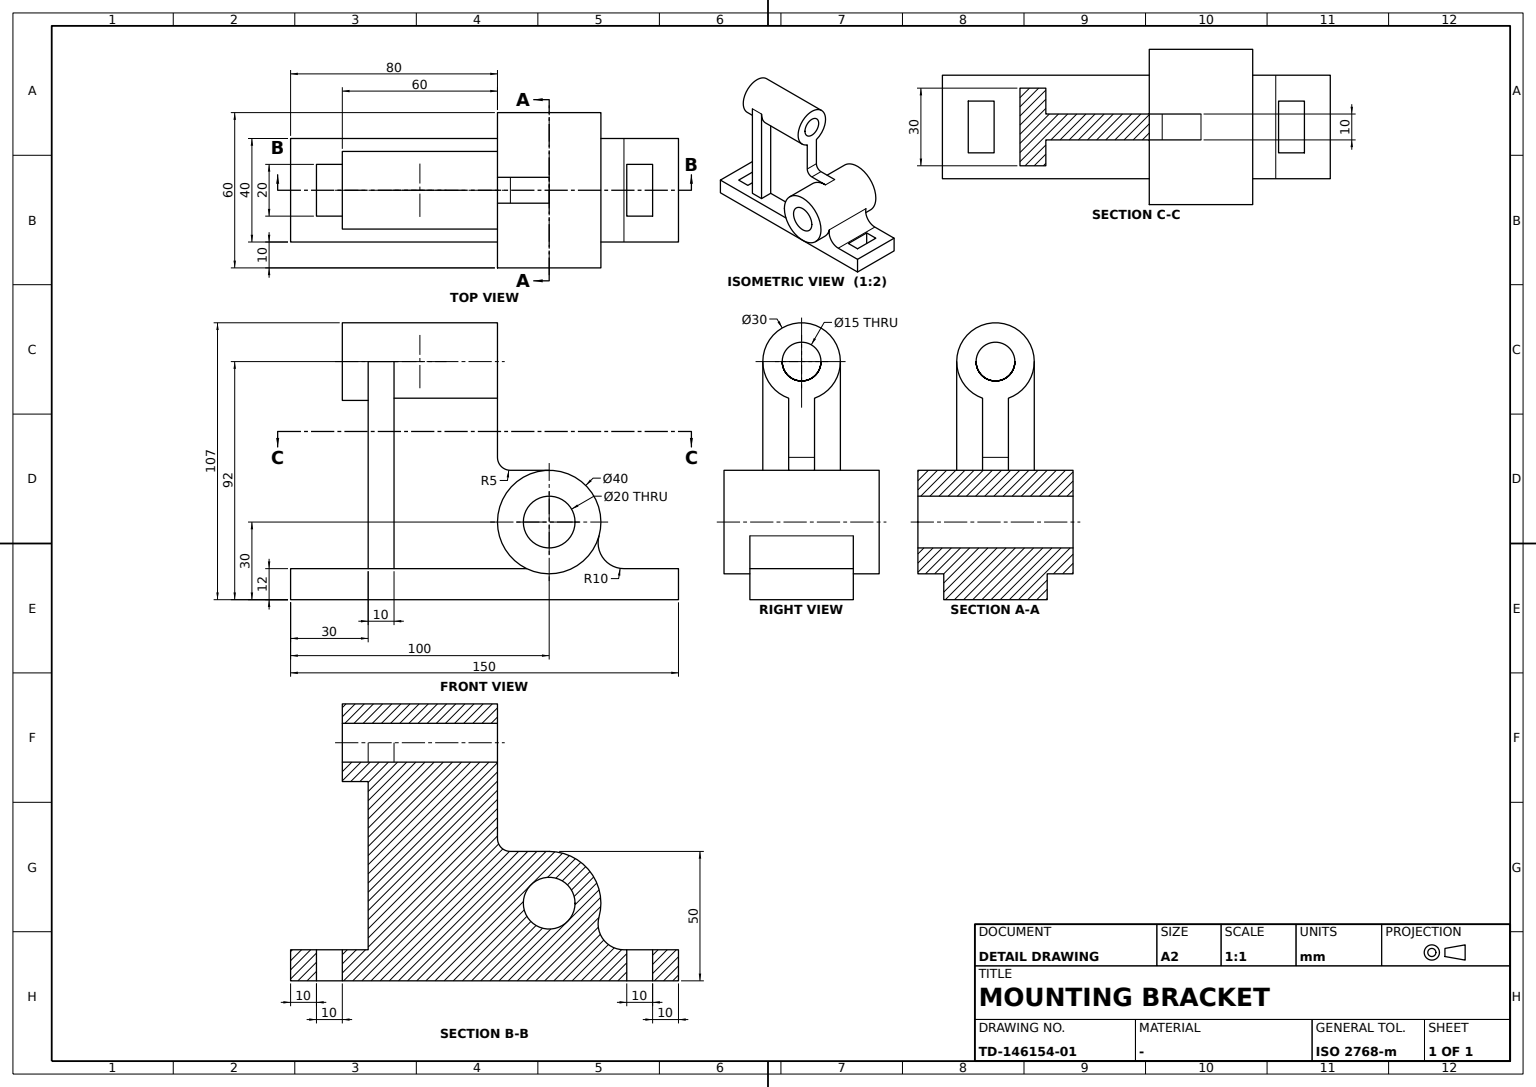
ISO-10303-21;
HEADER;
FILE_DESCRIPTION((''),'2;1');
FILE_NAME('','',(''),(''),'','','');
FILE_SCHEMA(('AUTOMOTIVE_DESIGN'));
ENDSEC;
DATA;
#1=APPLICATION_CONTEXT('');
#2=PRODUCT_CONTEXT('',#1,'mechanical');
#3=PRODUCT('','','',(#2));
#4=PRODUCT_DEFINITION_FORMATION('','',#3);
#5=PRODUCT_DEFINITION_CONTEXT('',#1,'design');
#6=PRODUCT_DEFINITION('','',#4,#5);
#7=PRODUCT_DEFINITION_SHAPE('','',#6);
#8=(LENGTH_UNIT()NAMED_UNIT(*)SI_UNIT(.MILLI.,.METRE.));
#9=(NAMED_UNIT(*)PLANE_ANGLE_UNIT()SI_UNIT($,.RADIAN.));
#10=(NAMED_UNIT(*)SI_UNIT($,.STERADIAN.)SOLID_ANGLE_UNIT());
#11=UNCERTAINTY_MEASURE_WITH_UNIT(LENGTH_MEASURE(1.E-05),#8,'distance_accuracy_value','');
#12=(GEOMETRIC_REPRESENTATION_CONTEXT(3)GLOBAL_UNCERTAINTY_ASSIGNED_CONTEXT((#11))GLOBAL_UNIT_ASSIGNED_CONTEXT((#8,#9,#10))REPRESENTATION_CONTEXT('',''));
#13=CARTESIAN_POINT('',(20.,-8.717798,-18.));
#14=VERTEX_POINT('',#13);
#15=CARTESIAN_POINT('',(20.,-100.,-18.));
#16=VERTEX_POINT('',#15);
#17=CARTESIAN_POINT('',(20.,-54.358899,-18.));
#18=DIRECTION('',(0.,-1.,0.));
#19=VECTOR('',#18,1000.);
#20=LINE('',#17,#19);
#21=EDGE_CURVE('',#14,#16,#20,.T.);
#22=ORIENTED_EDGE('',*,*,#21,.T.);
#23=CARTESIAN_POINT('',(20.,-100.,-30.));
#24=VERTEX_POINT('',#23);
#25=CARTESIAN_POINT('',(20.,-100.,-24.));
#26=DIRECTION('',(0.,0.,-1.));
#27=VECTOR('',#26,1000.);
#28=LINE('',#25,#27);
#29=EDGE_CURVE('',#16,#24,#28,.T.);
#30=ORIENTED_EDGE('',*,*,#29,.T.);
#31=CARTESIAN_POINT('',(20.,50.,-30.));
#32=VERTEX_POINT('',#31);
#33=CARTESIAN_POINT('',(20.,-25.,-30.));
#34=DIRECTION('',(0.,1.,0.));
#35=VECTOR('',#34,1000.);
#36=LINE('',#33,#35);
#37=EDGE_CURVE('',#24,#32,#36,.T.);
#38=ORIENTED_EDGE('',*,*,#37,.T.);
#39=CARTESIAN_POINT('',(20.,50.,-18.));
#40=VERTEX_POINT('',#39);
#41=CARTESIAN_POINT('',(20.,50.,-24.));
#42=DIRECTION('',(0.,0.,1.));
#43=VECTOR('',#42,1000.);
#44=LINE('',#41,#43);
#45=EDGE_CURVE('',#32,#40,#44,.T.);
#46=ORIENTED_EDGE('',*,*,#45,.T.);
#47=CARTESIAN_POINT('',(20.,28.913665,-18.));
#48=VERTEX_POINT('',#47);
#49=CARTESIAN_POINT('',(20.,39.456832,-18.));
#50=LINE('',#49,#19);
#51=EDGE_CURVE('',#40,#48,#50,.T.);
#52=ORIENTED_EDGE('',*,*,#51,.T.);
#53=CARTESIAN_POINT('',(20.,19.275776,-5.333333));
#54=VERTEX_POINT('',#53);
#55=CARTESIAN_POINT('',(20.,28.913665,-8.));
#56=DIRECTION('',(-1.,0.,0.));
#57=AXIS2_PLACEMENT_3D('',#55,#56,#34);
#58=CIRCLE('',#57,10.);
#59=EDGE_CURVE('',#48,#54,#58,.T.);
#60=ORIENTED_EDGE('',*,*,#59,.T.);
#61=CARTESIAN_POINT('',(20.,0.,0.));
#62=DIRECTION('',(1.,0.,0.));
#63=AXIS2_PLACEMENT_3D('',#61,#62,#34);
#64=CIRCLE('',#63,20.);
#65=EDGE_CURVE('',#14,#54,#64,.T.);
#66=ORIENTED_EDGE('',*,*,#65,.F.);
#67=EDGE_LOOP('',(#22,#30,#38,#46,#52,#60,#66));
#68=FACE_OUTER_BOUND('',#67,.T.);
#69=PLANE('',#63);
#70=ADVANCED_FACE('',(#68),#69,.T.);
#71=CARTESIAN_POINT('',(15.,-70.,62.));
#72=VERTEX_POINT('',#71);
#73=CARTESIAN_POINT('',(-15.,-70.,62.));
#74=VERTEX_POINT('',#73);
#75=CARTESIAN_POINT('',(0.,-70.,62.));
#76=AXIS2_PLACEMENT_3D('',#75,#34,#26);
#77=CIRCLE('',#76,15.);
#78=EDGE_CURVE('',#72,#74,#77,.T.);
#79=ORIENTED_EDGE('',*,*,#78,.T.);
#80=CARTESIAN_POINT('',(-15.,-70.,-18.));
#81=VERTEX_POINT('',#80);
#82=CARTESIAN_POINT('',(-15.,-70.,22.));
#83=LINE('',#82,#27);
#84=EDGE_CURVE('',#74,#81,#83,.T.);
#85=ORIENTED_EDGE('',*,*,#84,.T.);
#86=CARTESIAN_POINT('',(15.,-70.,-18.));
#87=VERTEX_POINT('',#86);
#88=CARTESIAN_POINT('',(0.,-70.,-18.));
#89=VECTOR('',#56,1000.);
#90=LINE('',#88,#89);
#91=EDGE_CURVE('',#87,#81,#90,.T.);
#92=ORIENTED_EDGE('',*,*,#91,.F.);
#93=CARTESIAN_POINT('',(15.,-70.,22.));
#94=LINE('',#93,#27);
#95=EDGE_CURVE('',#72,#87,#94,.T.);
#96=ORIENTED_EDGE('',*,*,#95,.F.);
#97=EDGE_LOOP('',(#79,#85,#92,#96));
#98=FACE_OUTER_BOUND('',#97,.T.);
#99=CARTESIAN_POINT('',(20.,-70.,62.));
#100=AXIS2_PLACEMENT_3D('',#99,#34,#26);
#101=PLANE('',#100);
#102=ADVANCED_FACE('',(#98),#101,.F.);
#103=CARTESIAN_POINT('',(-10.,30.,-18.));
#104=VERTEX_POINT('',#103);
#105=CARTESIAN_POINT('',(10.,30.,-18.));
#106=VERTEX_POINT('',#105);
#107=CARTESIAN_POINT('',(0.,30.,-18.));
#108=VECTOR('',#62,1000.);
#109=LINE('',#107,#108);
#110=EDGE_CURVE('',#104,#106,#109,.T.);
#111=ORIENTED_EDGE('',*,*,#110,.F.);
#112=CARTESIAN_POINT('',(-10.,40.,-18.));
#113=VERTEX_POINT('',#112);
#114=CARTESIAN_POINT('',(-10.,35.,-18.));
#115=LINE('',#114,#19);
#116=EDGE_CURVE('',#113,#104,#115,.T.);
#117=ORIENTED_EDGE('',*,*,#116,.F.);
#118=CARTESIAN_POINT('',(10.,40.,-18.));
#119=VERTEX_POINT('',#118);
#120=CARTESIAN_POINT('',(0.,40.,-18.));
#121=LINE('',#120,#89);
#122=EDGE_CURVE('',#119,#113,#121,.T.);
#123=ORIENTED_EDGE('',*,*,#122,.F.);
#124=CARTESIAN_POINT('',(10.,35.,-18.));
#125=LINE('',#124,#35);
#126=EDGE_CURVE('',#106,#119,#125,.T.);
#127=ORIENTED_EDGE('',*,*,#126,.F.);
#128=EDGE_LOOP('',(#111,#117,#123,#127));
#129=FACE_BOUND('',#128,.T.);
#130=CARTESIAN_POINT('',(-20.,50.,-18.));
#131=VERTEX_POINT('',#130);
#132=CARTESIAN_POINT('',(0.,50.,-18.));
#133=LINE('',#132,#108);
#134=EDGE_CURVE('',#131,#40,#133,.T.);
#135=ORIENTED_EDGE('',*,*,#134,.F.);
#136=CARTESIAN_POINT('',(-20.,28.913665,-18.));
#137=VERTEX_POINT('',#136);
#138=CARTESIAN_POINT('',(-20.,39.456832,-18.));
#139=LINE('',#138,#19);
#140=EDGE_CURVE('',#131,#137,#139,.T.);
#141=ORIENTED_EDGE('',*,*,#140,.T.);
#142=CARTESIAN_POINT('',(0.,28.913665,-18.));
#143=LINE('',#142,#108);
#144=EDGE_CURVE('',#137,#48,#143,.T.);
#145=ORIENTED_EDGE('',*,*,#144,.T.);
#146=ORIENTED_EDGE('',*,*,#51,.F.);
#147=EDGE_LOOP('',(#135,#141,#145,#146));
#148=FACE_OUTER_BOUND('',#147,.T.);
#149=AXIS2_PLACEMENT_3D('',#142,#26,#34);
#150=PLANE('',#149);
#151=ADVANCED_FACE('',(#129,#148),#150,.F.);
#152=CARTESIAN_POINT('',(10.,30.,-30.));
#153=VERTEX_POINT('',#152);
#154=CARTESIAN_POINT('',(-10.,30.,-30.));
#155=VERTEX_POINT('',#154);
#156=CARTESIAN_POINT('',(0.,30.,-30.));
#157=LINE('',#156,#89);
#158=EDGE_CURVE('',#153,#155,#157,.T.);
#159=ORIENTED_EDGE('',*,*,#158,.T.);
#160=CARTESIAN_POINT('',(-10.,30.,-24.));
#161=LINE('',#160,#27);
#162=EDGE_CURVE('',#104,#155,#161,.T.);
#163=ORIENTED_EDGE('',*,*,#162,.F.);
#164=ORIENTED_EDGE('',*,*,#110,.T.);
#165=CARTESIAN_POINT('',(10.,30.,-24.));
#166=LINE('',#165,#27);
#167=EDGE_CURVE('',#106,#153,#166,.T.);
#168=ORIENTED_EDGE('',*,*,#167,.T.);
#169=EDGE_LOOP('',(#159,#163,#164,#168));
#170=FACE_OUTER_BOUND('',#169,.T.);
#171=AXIS2_PLACEMENT_3D('',#105,#18,#56);
#172=PLANE('',#171);
#173=ADVANCED_FACE('',(#170),#172,.F.);
#174=CARTESIAN_POINT('',(-30.,10.,0.));
#175=VERTEX_POINT('',#174);
#176=CARTESIAN_POINT('',(-30.,-10.,0.));
#177=VERTEX_POINT('',#176);
#178=CARTESIAN_POINT('',(-30.,0.,0.));
#179=AXIS2_PLACEMENT_3D('',#178,#62,#34);
#180=CIRCLE('',#179,10.);
#181=EDGE_CURVE('',#175,#177,#180,.T.);
#182=ORIENTED_EDGE('',*,*,#181,.T.);
#183=EDGE_CURVE('',#177,#175,#180,.T.);
#184=ORIENTED_EDGE('',*,*,#183,.T.);
#185=EDGE_LOOP('',(#182,#184));
#186=FACE_BOUND('',#185,.T.);
#187=CARTESIAN_POINT('',(-30.,20.,0.));
#188=VERTEX_POINT('',#187);
#189=CARTESIAN_POINT('',(-30.,-20.,0.));
#190=VERTEX_POINT('',#189);
#191=CIRCLE('',#179,20.);
#192=EDGE_CURVE('',#188,#190,#191,.T.);
#193=ORIENTED_EDGE('',*,*,#192,.F.);
#194=CARTESIAN_POINT('',(-30.,19.275776,-5.333333));
#195=VERTEX_POINT('',#194);
#196=EDGE_CURVE('',#195,#188,#191,.T.);
#197=ORIENTED_EDGE('',*,*,#196,.F.);
#198=CARTESIAN_POINT('',(-30.,-8.717798,-18.));
#199=VERTEX_POINT('',#198);
#200=EDGE_CURVE('',#199,#195,#191,.T.);
#201=ORIENTED_EDGE('',*,*,#200,.F.);
#202=EDGE_CURVE('',#190,#199,#191,.T.);
#203=ORIENTED_EDGE('',*,*,#202,.F.);
#204=EDGE_LOOP('',(#193,#197,#201,#203));
#205=FACE_OUTER_BOUND('',#204,.T.);
#206=PLANE('',#179);
#207=ADVANCED_FACE('',(#186,#205),#206,.F.);
#208=CARTESIAN_POINT('',(-20.,19.275776,-5.333333));
#209=VERTEX_POINT('',#208);
#210=CARTESIAN_POINT('',(0.,19.275776,-5.333333));
#211=LINE('',#210,#108);
#212=EDGE_CURVE('',#209,#54,#211,.T.);
#213=ORIENTED_EDGE('',*,*,#212,.T.);
#214=ORIENTED_EDGE('',*,*,#59,.F.);
#215=ORIENTED_EDGE('',*,*,#144,.F.);
#216=CARTESIAN_POINT('',(-20.,28.913665,-8.));
#217=AXIS2_PLACEMENT_3D('',#216,#56,#34);
#218=CIRCLE('',#217,10.);
#219=EDGE_CURVE('',#137,#209,#218,.T.);
#220=ORIENTED_EDGE('',*,*,#219,.T.);
#221=EDGE_LOOP('',(#213,#214,#215,#220));
#222=FACE_OUTER_BOUND('',#221,.T.);
#223=CARTESIAN_POINT('',(0.,28.913665,-8.));
#224=AXIS2_PLACEMENT_3D('',#223,#56,#34);
#225=CYLINDRICAL_SURFACE('',#224,10.);
#226=ADVANCED_FACE('',(#222),#225,.F.);
#227=CARTESIAN_POINT('',(-15.,-60.,-18.));
#228=VERTEX_POINT('',#227);
#229=CARTESIAN_POINT('',(-15.,-65.,-18.));
#230=LINE('',#229,#35);
#231=EDGE_CURVE('',#81,#228,#230,.T.);
#232=ORIENTED_EDGE('',*,*,#231,.F.);
#233=ORIENTED_EDGE('',*,*,#84,.F.);
#234=CARTESIAN_POINT('',(-15.,-60.,62.));
#235=VERTEX_POINT('',#234);
#236=CARTESIAN_POINT('',(-15.,-65.,62.));
#237=LINE('',#236,#19);
#238=EDGE_CURVE('',#235,#74,#237,.T.);
#239=ORIENTED_EDGE('',*,*,#238,.F.);
#240=CARTESIAN_POINT('',(-15.,-60.,22.));
#241=LINE('',#240,#43);
#242=EDGE_CURVE('',#228,#235,#241,.T.);
#243=ORIENTED_EDGE('',*,*,#242,.F.);
#244=EDGE_LOOP('',(#232,#233,#239,#243));
#245=FACE_OUTER_BOUND('',#244,.T.);
#246=CARTESIAN_POINT('',(-15.,0.,0.));
#247=AXIS2_PLACEMENT_3D('',#246,#62,#34);
#248=PLANE('',#247);
#249=ADVANCED_FACE('',(#245),#248,.F.);
#250=CARTESIAN_POINT('',(5.,-20.,0.));
#251=VERTEX_POINT('',#250);
#252=CARTESIAN_POINT('',(5.,-8.717798,-18.));
#253=VERTEX_POINT('',#252);
#254=CARTESIAN_POINT('',(5.,0.,0.));
#255=AXIS2_PLACEMENT_3D('',#254,#62,#34);
#256=CIRCLE('',#255,20.);
#257=EDGE_CURVE('',#251,#253,#256,.T.);
#258=ORIENTED_EDGE('',*,*,#257,.T.);
#259=CARTESIAN_POINT('',(12.5,-8.717798,-18.));
#260=LINE('',#259,#108);
#261=EDGE_CURVE('',#253,#14,#260,.T.);
#262=ORIENTED_EDGE('',*,*,#261,.T.);
#263=CARTESIAN_POINT('',(30.,-8.717798,-18.));
#264=VERTEX_POINT('',#263);
#265=CARTESIAN_POINT('',(0.,-8.717798,-18.));
#266=LINE('',#265,#108);
#267=EDGE_CURVE('',#14,#264,#266,.T.);
#268=ORIENTED_EDGE('',*,*,#267,.T.);
#269=CARTESIAN_POINT('',(30.,-20.,0.));
#270=VERTEX_POINT('',#269);
#271=CARTESIAN_POINT('',(30.,0.,0.));
#272=AXIS2_PLACEMENT_3D('',#271,#62,#34);
#273=CIRCLE('',#272,20.);
#274=EDGE_CURVE('',#270,#264,#273,.T.);
#275=ORIENTED_EDGE('',*,*,#274,.F.);
#276=CARTESIAN_POINT('',(0.,-20.,0.));
#277=LINE('',#276,#89);
#278=EDGE_CURVE('',#270,#251,#277,.T.);
#279=ORIENTED_EDGE('',*,*,#278,.T.);
#280=EDGE_LOOP('',(#258,#262,#268,#275,#279));
#281=FACE_OUTER_BOUND('',#280,.T.);
#282=CARTESIAN_POINT('',(0.,0.,0.));
#283=AXIS2_PLACEMENT_3D('',#282,#56,#34);
#284=CYLINDRICAL_SURFACE('',#283,20.);
#285=ADVANCED_FACE('',(#281),#284,.T.);
#286=CARTESIAN_POINT('',(-20.,50.,-30.));
#287=VERTEX_POINT('',#286);
#288=CARTESIAN_POINT('',(0.,50.,-30.));
#289=LINE('',#288,#108);
#290=EDGE_CURVE('',#287,#32,#289,.T.);
#291=ORIENTED_EDGE('',*,*,#290,.F.);
#292=CARTESIAN_POINT('',(-20.,50.,-24.));
#293=LINE('',#292,#43);
#294=EDGE_CURVE('',#287,#131,#293,.T.);
#295=ORIENTED_EDGE('',*,*,#294,.T.);
#296=ORIENTED_EDGE('',*,*,#134,.T.);
#297=ORIENTED_EDGE('',*,*,#45,.F.);
#298=EDGE_LOOP('',(#291,#295,#296,#297));
#299=FACE_OUTER_BOUND('',#298,.T.);
#300=AXIS2_PLACEMENT_3D('',#132,#18,#26);
#301=PLANE('',#300);
#302=ADVANCED_FACE('',(#299),#301,.F.);
#303=ORIENTED_EDGE('',*,*,#181,.F.);
#304=CARTESIAN_POINT('',(30.,10.,0.));
#305=VERTEX_POINT('',#304);
#306=CARTESIAN_POINT('',(0.,10.,0.));
#307=LINE('',#306,#108);
#308=EDGE_CURVE('',#175,#305,#307,.T.);
#309=ORIENTED_EDGE('',*,*,#308,.T.);
#310=CARTESIAN_POINT('',(30.,-10.,0.));
#311=VERTEX_POINT('',#310);
#312=CIRCLE('',#272,10.);
#313=EDGE_CURVE('',#305,#311,#312,.T.);
#314=ORIENTED_EDGE('',*,*,#313,.T.);
#315=CARTESIAN_POINT('',(0.,-10.,0.));
#316=LINE('',#315,#108);
#317=EDGE_CURVE('',#177,#311,#316,.T.);
#318=ORIENTED_EDGE('',*,*,#317,.F.);
#319=EDGE_LOOP('',(#303,#309,#314,#318));
#320=FACE_OUTER_BOUND('',#319,.T.);
#321=CYLINDRICAL_SURFACE('',#283,10.);
#322=ADVANCED_FACE('',(#320),#321,.F.);
#323=CARTESIAN_POINT('',(-20.,-100.,-30.));
#324=VERTEX_POINT('',#323);
#325=CARTESIAN_POINT('',(-20.,-25.,-30.));
#326=LINE('',#325,#35);
#327=EDGE_CURVE('',#324,#287,#326,.T.);
#328=ORIENTED_EDGE('',*,*,#327,.F.);
#329=CARTESIAN_POINT('',(-20.,-100.,-18.));
#330=VERTEX_POINT('',#329);
#331=CARTESIAN_POINT('',(-20.,-100.,-24.));
#332=LINE('',#331,#27);
#333=EDGE_CURVE('',#330,#324,#332,.T.);
#334=ORIENTED_EDGE('',*,*,#333,.F.);
#335=CARTESIAN_POINT('',(-20.,-8.717798,-18.));
#336=VERTEX_POINT('',#335);
#337=CARTESIAN_POINT('',(-20.,-54.358899,-18.));
#338=LINE('',#337,#19);
#339=EDGE_CURVE('',#336,#330,#338,.T.);
#340=ORIENTED_EDGE('',*,*,#339,.F.);
#341=CARTESIAN_POINT('',(-20.,0.,0.));
#342=AXIS2_PLACEMENT_3D('',#341,#62,#34);
#343=CIRCLE('',#342,20.);
#344=EDGE_CURVE('',#336,#209,#343,.T.);
#345=ORIENTED_EDGE('',*,*,#344,.T.);
#346=ORIENTED_EDGE('',*,*,#219,.F.);
#347=ORIENTED_EDGE('',*,*,#140,.F.);
#348=ORIENTED_EDGE('',*,*,#294,.F.);
#349=EDGE_LOOP('',(#328,#334,#340,#345,#346,#347,#348));
#350=FACE_OUTER_BOUND('',#349,.T.);
#351=PLANE('',#342);
#352=ADVANCED_FACE('',(#350),#351,.F.);
#353=CARTESIAN_POINT('',(-10.,-90.,-18.));
#354=VERTEX_POINT('',#353);
#355=CARTESIAN_POINT('',(-10.,-90.,-30.));
#356=VERTEX_POINT('',#355);
#357=CARTESIAN_POINT('',(-10.,-90.,-24.));
#358=LINE('',#357,#27);
#359=EDGE_CURVE('',#354,#356,#358,.T.);
#360=ORIENTED_EDGE('',*,*,#359,.F.);
#361=CARTESIAN_POINT('',(10.,-90.,-18.));
#362=VERTEX_POINT('',#361);
#363=CARTESIAN_POINT('',(0.,-90.,-18.));
#364=LINE('',#363,#108);
#365=EDGE_CURVE('',#354,#362,#364,.T.);
#366=ORIENTED_EDGE('',*,*,#365,.T.);
#367=CARTESIAN_POINT('',(10.,-90.,-30.));
#368=VERTEX_POINT('',#367);
#369=CARTESIAN_POINT('',(10.,-90.,-24.));
#370=LINE('',#369,#27);
#371=EDGE_CURVE('',#362,#368,#370,.T.);
#372=ORIENTED_EDGE('',*,*,#371,.T.);
#373=CARTESIAN_POINT('',(0.,-90.,-30.));
#374=LINE('',#373,#89);
#375=EDGE_CURVE('',#368,#356,#374,.T.);
#376=ORIENTED_EDGE('',*,*,#375,.T.);
#377=EDGE_LOOP('',(#360,#366,#372,#376));
#378=FACE_OUTER_BOUND('',#377,.T.);
#379=AXIS2_PLACEMENT_3D('',#361,#18,#56);
#380=PLANE('',#379);
#381=ADVANCED_FACE('',(#378),#380,.F.);
#382=CARTESIAN_POINT('',(0.,-100.,-18.));
#383=LINE('',#382,#108);
#384=EDGE_CURVE('',#330,#16,#383,.T.);
#385=ORIENTED_EDGE('',*,*,#384,.F.);
#386=ORIENTED_EDGE('',*,*,#333,.T.);
#387=CARTESIAN_POINT('',(0.,-100.,-30.));
#388=LINE('',#387,#108);
#389=EDGE_CURVE('',#324,#24,#388,.T.);
#390=ORIENTED_EDGE('',*,*,#389,.T.);
#391=ORIENTED_EDGE('',*,*,#29,.F.);
#392=EDGE_LOOP('',(#385,#386,#390,#391));
#393=FACE_OUTER_BOUND('',#392,.T.);
#394=AXIS2_PLACEMENT_3D('',#387,#34,#42);
#395=PLANE('',#394);
#396=ADVANCED_FACE('',(#393),#395,.F.);
#397=CARTESIAN_POINT('',(-5.,-20.,47.));
#398=VERTEX_POINT('',#397);
#399=CARTESIAN_POINT('',(-5.,-20.,25.));
#400=VERTEX_POINT('',#399);
#401=CARTESIAN_POINT('',(-5.,-20.,36.));
#402=LINE('',#401,#27);
#403=EDGE_CURVE('',#398,#400,#402,.T.);
#404=ORIENTED_EDGE('',*,*,#403,.F.);
#405=CARTESIAN_POINT('',(5.,-20.,47.));
#406=VERTEX_POINT('',#405);
#407=CARTESIAN_POINT('',(0.,-20.,47.));
#408=LINE('',#407,#108);
#409=EDGE_CURVE('',#398,#406,#408,.T.);
#410=ORIENTED_EDGE('',*,*,#409,.T.);
#411=CARTESIAN_POINT('',(5.,-20.,25.));
#412=VERTEX_POINT('',#411);
#413=CARTESIAN_POINT('',(5.,-20.,36.));
#414=LINE('',#413,#27);
#415=EDGE_CURVE('',#406,#412,#414,.T.);
#416=ORIENTED_EDGE('',*,*,#415,.T.);
#417=CARTESIAN_POINT('',(0.,-20.,25.));
#418=LINE('',#417,#89);
#419=EDGE_CURVE('',#412,#400,#418,.T.);
#420=ORIENTED_EDGE('',*,*,#419,.T.);
#421=EDGE_LOOP('',(#404,#410,#416,#420));
#422=FACE_OUTER_BOUND('',#421,.T.);
#423=AXIS2_PLACEMENT_3D('',#276,#34,#56);
#424=PLANE('',#423);
#425=ADVANCED_FACE('',(#422),#424,.T.);
#426=CARTESIAN_POINT('',(7.5,-60.,62.));
#427=VERTEX_POINT('',#426);
#428=CARTESIAN_POINT('',(-7.5,-60.,62.));
#429=VERTEX_POINT('',#428);
#430=CARTESIAN_POINT('',(7.5,-60.,60.821903));
#431=CARTESIAN_POINT('',(7.268681,-60.,59.643806));
#432=CARTESIAN_POINT('',(6.805815,-60.,58.526347));
#433=CARTESIAN_POINT('',(5.466868,-60.,56.533132));
#434=CARTESIAN_POINT('',(3.473653,-60.,55.194185));
#435=CARTESIAN_POINT('',(2.356194,-60.,54.731319));
#436=CARTESIAN_POINT('',(0.,-60.,54.268681));
#437=CARTESIAN_POINT('',(-2.356194,-60.,54.731319));
#438=CARTESIAN_POINT('',(-3.473653,-60.,55.194185));
#439=CARTESIAN_POINT('',(-5.466868,-60.,56.533132));
#440=CARTESIAN_POINT('',(-6.805815,-60.,58.526347));
#441=CARTESIAN_POINT('',(-7.268681,-60.,59.643806));
#442=CARTESIAN_POINT('',(-7.5,-60.,60.821903));
#443=B_SPLINE_CURVE_WITH_KNOTS('',5,(#426,#430,#431,#432,#433,#434,#435,#436,#437,#438,#439,#440,#441,#442,#428),.UNSPECIFIED.,.F.,.F.,(6,3,3,3,6),(0.,0.25,0.5,0.75,1.),.UNSPECIFIED.);
#444=EDGE_CURVE('',#427,#429,#443,.T.);
#445=ORIENTED_EDGE('',*,*,#444,.T.);
#446=CARTESIAN_POINT('',(-7.5,-70.,62.));
#447=VERTEX_POINT('',#446);
#448=CARTESIAN_POINT('',(-7.5,-80.66,62.));
#449=LINE('',#448,#19);
#450=EDGE_CURVE('',#429,#447,#449,.T.);
#451=ORIENTED_EDGE('',*,*,#450,.T.);
#452=CARTESIAN_POINT('',(7.5,-70.,62.));
#453=VERTEX_POINT('',#452);
#454=CARTESIAN_POINT('',(7.5,-70.,61.018252));
#455=CARTESIAN_POINT('',(7.304795,-70.,60.036891));
#456=CARTESIAN_POINT('',(6.553398,-70.,58.222858));
#457=CARTESIAN_POINT('',(5.997501,-70.,57.3909));
#458=CARTESIAN_POINT('',(4.6091,-70.,56.002499));
#459=CARTESIAN_POINT('',(3.777142,-70.,55.446602));
#460=CARTESIAN_POINT('',(1.963109,-70.,54.695205));
#461=CARTESIAN_POINT('',(0.981748,-70.,54.5));
#462=CARTESIAN_POINT('',(-0.981748,-70.,54.5));
#463=CARTESIAN_POINT('',(-1.963109,-70.,54.695205));
#464=CARTESIAN_POINT('',(-3.777142,-70.,55.446602));
#465=CARTESIAN_POINT('',(-4.6091,-70.,56.002499));
#466=CARTESIAN_POINT('',(-5.997501,-70.,57.3909));
#467=CARTESIAN_POINT('',(-6.553398,-70.,58.222858));
#468=CARTESIAN_POINT('',(-7.304795,-70.,60.036891));
#469=CARTESIAN_POINT('',(-7.5,-70.,61.018252));
#470=B_SPLINE_CURVE_WITH_KNOTS('',3,(#452,#454,#455,#456,#457,#458,#459,#460,#461,#462,#463,#464,#465,#466,#467,#468,#469,#446),.UNSPECIFIED.,.F.,.F.,(4,2,2,2,2,2,2,2,4),(0.,0.125,0.25,0.375,0.5,0.625,0.75,0.875,1.),.UNSPECIFIED.);
#471=EDGE_CURVE('',#453,#447,#470,.T.);
#472=ORIENTED_EDGE('',*,*,#471,.F.);
#473=CARTESIAN_POINT('',(7.5,-80.66,62.));
#474=LINE('',#473,#19);
#475=EDGE_CURVE('',#427,#453,#474,.T.);
#476=ORIENTED_EDGE('',*,*,#475,.F.);
#477=EDGE_LOOP('',(#445,#451,#472,#476));
#478=FACE_OUTER_BOUND('',#477,.T.);
#479=CARTESIAN_POINT('',(-7.5,-70.,60.821903));
#480=CARTESIAN_POINT('',(-7.268681,-70.,59.643806));
#481=CARTESIAN_POINT('',(-6.805815,-70.,58.526347));
#482=CARTESIAN_POINT('',(-5.466868,-70.,56.533132));
#483=CARTESIAN_POINT('',(-3.473653,-70.,55.194185));
#484=CARTESIAN_POINT('',(-2.356194,-70.,54.731319));
#485=CARTESIAN_POINT('',(0.,-70.,54.268681));
#486=CARTESIAN_POINT('',(2.356194,-70.,54.731319));
#487=CARTESIAN_POINT('',(3.473653,-70.,55.194185));
#488=CARTESIAN_POINT('',(5.466868,-70.,56.533132));
#489=CARTESIAN_POINT('',(6.805815,-70.,58.526347));
#490=CARTESIAN_POINT('',(7.268681,-70.,59.643806));
#491=CARTESIAN_POINT('',(7.5,-70.,60.821903));
#492=B_SPLINE_SURFACE_WITH_KNOTS('',5,1,((#428,#446),(#442,#479),(#441,#480),(#440,#481),(#439,#482),(#438,#483),(#437,#484),(#436,#485),(#435,#486),(#434,#487),(#433,#488),(#432,#489),(#431,#490),(#430,#491),(#426,#452)),.UNSPECIFIED.,.F.,.F.,.F.,(6,3,3,3,6),(2,2),(15.,20.890486225,26.780972451,32.671458676,38.561944902),(0.,10.),.UNSPECIFIED.);
#493=ADVANCED_FACE('',(#478),#492,.F.);
#494=CARTESIAN_POINT('',(-5.,-20.,0.));
#495=VERTEX_POINT('',#494);
#496=EDGE_CURVE('',#495,#190,#277,.T.);
#497=ORIENTED_EDGE('',*,*,#496,.T.);
#498=ORIENTED_EDGE('',*,*,#202,.T.);
#499=EDGE_CURVE('',#199,#336,#266,.T.);
#500=ORIENTED_EDGE('',*,*,#499,.T.);
#501=CARTESIAN_POINT('',(-5.,-8.717798,-18.));
#502=VERTEX_POINT('',#501);
#503=CARTESIAN_POINT('',(-12.5,-8.717798,-18.));
#504=LINE('',#503,#108);
#505=EDGE_CURVE('',#336,#502,#504,.T.);
#506=ORIENTED_EDGE('',*,*,#505,.T.);
#507=CARTESIAN_POINT('',(-5.,0.,0.));
#508=AXIS2_PLACEMENT_3D('',#507,#62,#34);
#509=CIRCLE('',#508,20.);
#510=EDGE_CURVE('',#495,#502,#509,.T.);
#511=ORIENTED_EDGE('',*,*,#510,.F.);
#512=EDGE_LOOP('',(#497,#498,#500,#506,#511));
#513=FACE_OUTER_BOUND('',#512,.T.);
#514=ADVANCED_FACE('',(#513),#284,.T.);
#515=CARTESIAN_POINT('',(-7.5,-80.,62.));
#516=VERTEX_POINT('',#515);
#517=CARTESIAN_POINT('',(7.5,-80.,62.));
#518=VERTEX_POINT('',#517);
#519=CARTESIAN_POINT('',(0.,-80.,62.));
#520=AXIS2_PLACEMENT_3D('',#519,#34,#56);
#521=CIRCLE('',#520,7.5);
#522=EDGE_CURVE('',#516,#518,#521,.T.);
#523=ORIENTED_EDGE('',*,*,#522,.T.);
#524=EDGE_CURVE('',#518,#516,#521,.T.);
#525=ORIENTED_EDGE('',*,*,#524,.T.);
#526=EDGE_LOOP('',(#523,#525));
#527=FACE_BOUND('',#526,.T.);
#528=CARTESIAN_POINT('',(-15.,-80.,62.));
#529=VERTEX_POINT('',#528);
#530=CARTESIAN_POINT('',(15.,-80.,62.));
#531=VERTEX_POINT('',#530);
#532=CIRCLE('',#520,15.);
#533=EDGE_CURVE('',#529,#531,#532,.T.);
#534=ORIENTED_EDGE('',*,*,#533,.F.);
#535=EDGE_CURVE('',#531,#529,#532,.T.);
#536=ORIENTED_EDGE('',*,*,#535,.F.);
#537=EDGE_LOOP('',(#534,#536));
#538=FACE_OUTER_BOUND('',#537,.T.);
#539=CARTESIAN_POINT('',(0.,-80.,0.));
#540=AXIS2_PLACEMENT_3D('',#539,#34,#56);
#541=PLANE('',#540);
#542=ADVANCED_FACE('',(#527,#538),#541,.F.);
#543=CARTESIAN_POINT('',(-15.,-20.,62.));
#544=VERTEX_POINT('',#543);
#545=CARTESIAN_POINT('',(-15.,-50.,62.));
#546=LINE('',#545,#19);
#547=EDGE_CURVE('',#544,#235,#546,.T.);
#548=ORIENTED_EDGE('',*,*,#547,.F.);
#549=CARTESIAN_POINT('',(-5.,-20.,47.857864));
#550=VERTEX_POINT('',#549);
#551=CARTESIAN_POINT('',(0.,-20.,62.));
#552=AXIS2_PLACEMENT_3D('',#551,#34,#56);
#553=CIRCLE('',#552,15.);
#554=EDGE_CURVE('',#550,#544,#553,.T.);
#555=ORIENTED_EDGE('',*,*,#554,.F.);
#556=CARTESIAN_POINT('',(-5.,-60.,47.857864));
#557=VERTEX_POINT('',#556);
#558=CARTESIAN_POINT('',(-5.,-40.,47.857864));
#559=LINE('',#558,#35);
#560=EDGE_CURVE('',#557,#550,#559,.T.);
#561=ORIENTED_EDGE('',*,*,#560,.F.);
#562=CARTESIAN_POINT('',(0.,-60.,62.));
#563=AXIS2_PLACEMENT_3D('',#562,#18,#42);
#564=CIRCLE('',#563,15.);
#565=EDGE_CURVE('',#235,#557,#564,.T.);
#566=ORIENTED_EDGE('',*,*,#565,.F.);
#567=EDGE_LOOP('',(#548,#555,#561,#566));
#568=FACE_OUTER_BOUND('',#567,.T.);
#569=CARTESIAN_POINT('',(0.,-50.,62.));
#570=AXIS2_PLACEMENT_3D('',#569,#18,#56);
#571=CYLINDRICAL_SURFACE('',#570,15.);
#572=ADVANCED_FACE('',(#568),#571,.T.);
#573=CARTESIAN_POINT('',(15.,-60.,-18.));
#574=VERTEX_POINT('',#573);
#575=CARTESIAN_POINT('',(5.,-60.,-18.));
#576=VERTEX_POINT('',#575);
#577=CARTESIAN_POINT('',(10.,-60.,-18.));
#578=LINE('',#577,#89);
#579=EDGE_CURVE('',#574,#576,#578,.T.);
#580=ORIENTED_EDGE('',*,*,#579,.T.);
#581=CARTESIAN_POINT('',(5.,-60.,47.857864));
#582=VERTEX_POINT('',#581);
#583=CARTESIAN_POINT('',(5.,-60.,14.928932));
#584=LINE('',#583,#43);
#585=EDGE_CURVE('',#576,#582,#584,.T.);
#586=ORIENTED_EDGE('',*,*,#585,.T.);
#587=CARTESIAN_POINT('',(15.,-60.,62.));
#588=VERTEX_POINT('',#587);
#589=EDGE_CURVE('',#582,#588,#564,.T.);
#590=ORIENTED_EDGE('',*,*,#589,.T.);
#591=CARTESIAN_POINT('',(15.,-60.,22.));
#592=LINE('',#591,#43);
#593=EDGE_CURVE('',#574,#588,#592,.T.);
#594=ORIENTED_EDGE('',*,*,#593,.F.);
#595=EDGE_LOOP('',(#580,#586,#590,#594));
#596=FACE_OUTER_BOUND('',#595,.T.);
#597=CARTESIAN_POINT('',(20.,-60.,-18.));
#598=AXIS2_PLACEMENT_3D('',#597,#18,#42);
#599=PLANE('',#598);
#600=ADVANCED_FACE('',(#596),#599,.F.);
#601=ORIENTED_EDGE('',*,*,#317,.T.);
#602=EDGE_CURVE('',#311,#305,#312,.T.);
#603=ORIENTED_EDGE('',*,*,#602,.T.);
#604=ORIENTED_EDGE('',*,*,#308,.F.);
#605=ORIENTED_EDGE('',*,*,#183,.F.);
#606=EDGE_LOOP('',(#601,#603,#604,#605));
#607=FACE_OUTER_BOUND('',#606,.T.);
#608=ADVANCED_FACE('',(#607),#321,.F.);
#609=CARTESIAN_POINT('',(-7.5,-50.,62.));
#610=LINE('',#609,#19);
#611=EDGE_CURVE('',#447,#516,#610,.T.);
#612=ORIENTED_EDGE('',*,*,#611,.T.);
#613=ORIENTED_EDGE('',*,*,#524,.F.);
#614=CARTESIAN_POINT('',(7.5,-50.,62.));
#615=LINE('',#614,#19);
#616=EDGE_CURVE('',#453,#518,#615,.T.);
#617=ORIENTED_EDGE('',*,*,#616,.F.);
#618=ORIENTED_EDGE('',*,*,#471,.T.);
#619=EDGE_LOOP('',(#612,#613,#617,#618));
#620=FACE_OUTER_BOUND('',#619,.T.);
#621=CYLINDRICAL_SURFACE('',#570,7.5);
#622=ADVANCED_FACE('',(#620),#621,.F.);
#623=EDGE_CURVE('',#195,#209,#211,.T.);
#624=ORIENTED_EDGE('',*,*,#623,.T.);
#625=ORIENTED_EDGE('',*,*,#344,.F.);
#626=ORIENTED_EDGE('',*,*,#499,.F.);
#627=ORIENTED_EDGE('',*,*,#200,.T.);
#628=EDGE_LOOP('',(#624,#625,#626,#627));
#629=FACE_OUTER_BOUND('',#628,.T.);
#630=ADVANCED_FACE('',(#629),#284,.T.);
#631=CARTESIAN_POINT('',(10.,-80.,-18.));
#632=VERTEX_POINT('',#631);
#633=CARTESIAN_POINT('',(10.,-80.,-30.));
#634=VERTEX_POINT('',#633);
#635=CARTESIAN_POINT('',(10.,-80.,-24.));
#636=LINE('',#635,#27);
#637=EDGE_CURVE('',#632,#634,#636,.T.);
#638=ORIENTED_EDGE('',*,*,#637,.F.);
#639=CARTESIAN_POINT('',(-10.,-80.,-18.));
#640=VERTEX_POINT('',#639);
#641=CARTESIAN_POINT('',(0.,-80.,-18.));
#642=LINE('',#641,#89);
#643=EDGE_CURVE('',#632,#640,#642,.T.);
#644=ORIENTED_EDGE('',*,*,#643,.T.);
#645=CARTESIAN_POINT('',(-10.,-80.,-30.));
#646=VERTEX_POINT('',#645);
#647=CARTESIAN_POINT('',(-10.,-80.,-24.));
#648=LINE('',#647,#27);
#649=EDGE_CURVE('',#640,#646,#648,.T.);
#650=ORIENTED_EDGE('',*,*,#649,.T.);
#651=CARTESIAN_POINT('',(0.,-80.,-30.));
#652=LINE('',#651,#89);
#653=EDGE_CURVE('',#634,#646,#652,.T.);
#654=ORIENTED_EDGE('',*,*,#653,.F.);
#655=EDGE_LOOP('',(#638,#644,#650,#654));
#656=FACE_OUTER_BOUND('',#655,.T.);
#657=ADVANCED_FACE('',(#656),#541,.F.);
#658=ORIENTED_EDGE('',*,*,#167,.F.);
#659=ORIENTED_EDGE('',*,*,#126,.T.);
#660=CARTESIAN_POINT('',(10.,40.,-30.));
#661=VERTEX_POINT('',#660);
#662=CARTESIAN_POINT('',(10.,40.,-24.));
#663=LINE('',#662,#27);
#664=EDGE_CURVE('',#119,#661,#663,.T.);
#665=ORIENTED_EDGE('',*,*,#664,.T.);
#666=CARTESIAN_POINT('',(10.,35.,-30.));
#667=LINE('',#666,#35);
#668=EDGE_CURVE('',#153,#661,#667,.T.);
#669=ORIENTED_EDGE('',*,*,#668,.F.);
#670=EDGE_LOOP('',(#658,#659,#665,#669));
#671=FACE_OUTER_BOUND('',#670,.T.);
#672=AXIS2_PLACEMENT_3D('',#361,#56,#34);
#673=PLANE('',#672);
#674=ADVANCED_FACE('',(#671),#673,.T.);
#675=ORIENTED_EDGE('',*,*,#267,.F.);
#676=ORIENTED_EDGE('',*,*,#65,.T.);
#677=CARTESIAN_POINT('',(30.,19.275776,-5.333333));
#678=VERTEX_POINT('',#677);
#679=EDGE_CURVE('',#54,#678,#211,.T.);
#680=ORIENTED_EDGE('',*,*,#679,.T.);
#681=EDGE_CURVE('',#264,#678,#273,.T.);
#682=ORIENTED_EDGE('',*,*,#681,.F.);
#683=EDGE_LOOP('',(#675,#676,#680,#682));
#684=FACE_OUTER_BOUND('',#683,.T.);
#685=ADVANCED_FACE('',(#684),#284,.T.);
#686=CARTESIAN_POINT('',(-5.,-15.,20.));
#687=VERTEX_POINT('',#686);
#688=CARTESIAN_POINT('',(-5.,0.,20.));
#689=VERTEX_POINT('',#688);
#690=CARTESIAN_POINT('',(-5.,-7.5,20.));
#691=LINE('',#690,#35);
#692=EDGE_CURVE('',#687,#689,#691,.T.);
#693=ORIENTED_EDGE('',*,*,#692,.F.);
#694=CARTESIAN_POINT('',(5.,-15.,20.));
#695=VERTEX_POINT('',#694);
#696=CARTESIAN_POINT('',(0.,-15.,20.));
#697=LINE('',#696,#89);
#698=EDGE_CURVE('',#695,#687,#697,.T.);
#699=ORIENTED_EDGE('',*,*,#698,.F.);
#700=CARTESIAN_POINT('',(5.,0.,20.));
#701=VERTEX_POINT('',#700);
#702=CARTESIAN_POINT('',(5.,-7.5,20.));
#703=LINE('',#702,#35);
#704=EDGE_CURVE('',#695,#701,#703,.T.);
#705=ORIENTED_EDGE('',*,*,#704,.T.);
#706=CARTESIAN_POINT('',(0.,0.,20.));
#707=LINE('',#706,#108);
#708=EDGE_CURVE('',#689,#701,#707,.T.);
#709=ORIENTED_EDGE('',*,*,#708,.F.);
#710=EDGE_LOOP('',(#693,#699,#705,#709));
#711=FACE_OUTER_BOUND('',#710,.T.);
#712=CARTESIAN_POINT('',(0.,-20.,20.));
#713=AXIS2_PLACEMENT_3D('',#712,#26,#34);
#714=PLANE('',#713);
#715=ADVANCED_FACE('',(#711),#714,.F.);
#716=ORIENTED_EDGE('',*,*,#122,.T.);
#717=CARTESIAN_POINT('',(-10.,40.,-30.));
#718=VERTEX_POINT('',#717);
#719=CARTESIAN_POINT('',(-10.,40.,-24.));
#720=LINE('',#719,#27);
#721=EDGE_CURVE('',#113,#718,#720,.T.);
#722=ORIENTED_EDGE('',*,*,#721,.T.);
#723=CARTESIAN_POINT('',(0.,40.,-30.));
#724=LINE('',#723,#108);
#725=EDGE_CURVE('',#718,#661,#724,.T.);
#726=ORIENTED_EDGE('',*,*,#725,.T.);
#727=ORIENTED_EDGE('',*,*,#664,.F.);
#728=EDGE_LOOP('',(#716,#722,#726,#727));
#729=FACE_OUTER_BOUND('',#728,.T.);
#730=AXIS2_PLACEMENT_3D('',#112,#34,#62);
#731=PLANE('',#730);
#732=ADVANCED_FACE('',(#729),#731,.F.);
#733=ORIENTED_EDGE('',*,*,#375,.F.);
#734=CARTESIAN_POINT('',(10.,-85.,-30.));
#735=LINE('',#734,#35);
#736=EDGE_CURVE('',#368,#634,#735,.T.);
#737=ORIENTED_EDGE('',*,*,#736,.T.);
#738=ORIENTED_EDGE('',*,*,#653,.T.);
#739=CARTESIAN_POINT('',(-10.,-85.,-30.));
#740=LINE('',#739,#19);
#741=EDGE_CURVE('',#646,#356,#740,.T.);
#742=ORIENTED_EDGE('',*,*,#741,.T.);
#743=EDGE_LOOP('',(#733,#737,#738,#742));
#744=FACE_BOUND('',#743,.T.);
#745=ORIENTED_EDGE('',*,*,#37,.F.);
#746=ORIENTED_EDGE('',*,*,#389,.F.);
#747=ORIENTED_EDGE('',*,*,#327,.T.);
#748=ORIENTED_EDGE('',*,*,#290,.T.);
#749=EDGE_LOOP('',(#745,#746,#747,#748));
#750=FACE_OUTER_BOUND('',#749,.T.);
#751=ORIENTED_EDGE('',*,*,#725,.F.);
#752=CARTESIAN_POINT('',(-10.,35.,-30.));
#753=LINE('',#752,#19);
#754=EDGE_CURVE('',#718,#155,#753,.T.);
#755=ORIENTED_EDGE('',*,*,#754,.T.);
#756=ORIENTED_EDGE('',*,*,#158,.F.);
#757=ORIENTED_EDGE('',*,*,#668,.T.);
#758=EDGE_LOOP('',(#751,#755,#756,#757));
#759=FACE_BOUND('',#758,.T.);
#760=AXIS2_PLACEMENT_3D('',#288,#42,#18);
#761=PLANE('',#760);
#762=ADVANCED_FACE('',(#744,#750,#759),#761,.F.);
#763=CARTESIAN_POINT('',(-5.,-60.,-18.));
#764=VERTEX_POINT('',#763);
#765=CARTESIAN_POINT('',(-10.,-60.,-18.));
#766=LINE('',#765,#89);
#767=EDGE_CURVE('',#764,#228,#766,.T.);
#768=ORIENTED_EDGE('',*,*,#767,.T.);
#769=ORIENTED_EDGE('',*,*,#242,.T.);
#770=ORIENTED_EDGE('',*,*,#565,.T.);
#771=CARTESIAN_POINT('',(-5.,-60.,14.928932));
#772=LINE('',#771,#43);
#773=EDGE_CURVE('',#764,#557,#772,.T.);
#774=ORIENTED_EDGE('',*,*,#773,.F.);
#775=EDGE_LOOP('',(#768,#769,#770,#774));
#776=FACE_OUTER_BOUND('',#775,.T.);
#777=ADVANCED_FACE('',(#776),#599,.F.);
#778=ORIENTED_EDGE('',*,*,#643,.F.);
#779=CARTESIAN_POINT('',(10.,-85.,-18.));
#780=LINE('',#779,#35);
#781=EDGE_CURVE('',#362,#632,#780,.T.);
#782=ORIENTED_EDGE('',*,*,#781,.F.);
#783=ORIENTED_EDGE('',*,*,#365,.F.);
#784=CARTESIAN_POINT('',(-10.,-85.,-18.));
#785=LINE('',#784,#19);
#786=EDGE_CURVE('',#640,#354,#785,.T.);
#787=ORIENTED_EDGE('',*,*,#786,.F.);
#788=EDGE_LOOP('',(#778,#782,#783,#787));
#789=FACE_BOUND('',#788,.T.);
#790=ORIENTED_EDGE('',*,*,#384,.T.);
#791=ORIENTED_EDGE('',*,*,#21,.F.);
#792=ORIENTED_EDGE('',*,*,#261,.F.);
#793=CARTESIAN_POINT('',(5.,-34.358899,-18.));
#794=LINE('',#793,#35);
#795=EDGE_CURVE('',#576,#253,#794,.T.);
#796=ORIENTED_EDGE('',*,*,#795,.F.);
#797=ORIENTED_EDGE('',*,*,#579,.F.);
#798=CARTESIAN_POINT('',(15.,-65.,-18.));
#799=LINE('',#798,#35);
#800=EDGE_CURVE('',#87,#574,#799,.T.);
#801=ORIENTED_EDGE('',*,*,#800,.F.);
#802=ORIENTED_EDGE('',*,*,#91,.T.);
#803=ORIENTED_EDGE('',*,*,#231,.T.);
#804=ORIENTED_EDGE('',*,*,#767,.F.);
#805=CARTESIAN_POINT('',(-5.,-34.358899,-18.));
#806=LINE('',#805,#35);
#807=EDGE_CURVE('',#764,#502,#806,.T.);
#808=ORIENTED_EDGE('',*,*,#807,.T.);
#809=ORIENTED_EDGE('',*,*,#505,.F.);
#810=ORIENTED_EDGE('',*,*,#339,.T.);
#811=EDGE_LOOP('',(#790,#791,#792,#796,#797,#801,#802,#803,#804,#808,#809,#810));
#812=FACE_OUTER_BOUND('',#811,.T.);
#813=ADVANCED_FACE('',(#789,#812),#150,.F.);
#814=CARTESIAN_POINT('',(15.,-50.,62.));
#815=LINE('',#814,#19);
#816=EDGE_CURVE('',#72,#531,#815,.T.);
#817=ORIENTED_EDGE('',*,*,#816,.T.);
#818=ORIENTED_EDGE('',*,*,#535,.T.);
#819=EDGE_CURVE('',#74,#529,#546,.T.);
#820=ORIENTED_EDGE('',*,*,#819,.F.);
#821=ORIENTED_EDGE('',*,*,#78,.F.);
#822=EDGE_LOOP('',(#817,#818,#820,#821));
#823=FACE_OUTER_BOUND('',#822,.T.);
#824=ADVANCED_FACE('',(#823),#571,.T.);
#825=EDGE_CURVE('',#701,#251,#256,.T.);
#826=ORIENTED_EDGE('',*,*,#825,.F.);
#827=ORIENTED_EDGE('',*,*,#704,.F.);
#828=CARTESIAN_POINT('',(5.,-15.,25.));
#829=AXIS2_PLACEMENT_3D('',#828,#56,#34);
#830=CIRCLE('',#829,5.);
#831=EDGE_CURVE('',#695,#412,#830,.T.);
#832=ORIENTED_EDGE('',*,*,#831,.T.);
#833=ORIENTED_EDGE('',*,*,#415,.F.);
#834=CARTESIAN_POINT('',(5.,-20.,47.857864));
#835=VERTEX_POINT('',#834);
#836=CARTESIAN_POINT('',(5.,-20.,47.428932));
#837=LINE('',#836,#27);
#838=EDGE_CURVE('',#835,#406,#837,.T.);
#839=ORIENTED_EDGE('',*,*,#838,.F.);
#840=CARTESIAN_POINT('',(5.,-40.,47.857864));
#841=LINE('',#840,#35);
#842=EDGE_CURVE('',#582,#835,#841,.T.);
#843=ORIENTED_EDGE('',*,*,#842,.F.);
#844=ORIENTED_EDGE('',*,*,#585,.F.);
#845=ORIENTED_EDGE('',*,*,#795,.T.);
#846=ORIENTED_EDGE('',*,*,#257,.F.);
#847=EDGE_LOOP('',(#826,#827,#832,#833,#839,#843,#844,#845,#846));
#848=FACE_OUTER_BOUND('',#847,.T.);
#849=PLANE('',#255);
#850=ADVANCED_FACE('',(#848),#849,.T.);
#851=ORIENTED_EDGE('',*,*,#698,.T.);
#852=CARTESIAN_POINT('',(-5.,-15.,25.));
#853=AXIS2_PLACEMENT_3D('',#852,#62,#34);
#854=CIRCLE('',#853,5.);
#855=EDGE_CURVE('',#400,#687,#854,.T.);
#856=ORIENTED_EDGE('',*,*,#855,.F.);
#857=ORIENTED_EDGE('',*,*,#419,.F.);
#858=ORIENTED_EDGE('',*,*,#831,.F.);
#859=EDGE_LOOP('',(#851,#856,#857,#858));
#860=FACE_OUTER_BOUND('',#859,.T.);
#861=CARTESIAN_POINT('',(0.,-15.,25.));
#862=AXIS2_PLACEMENT_3D('',#861,#56,#18);
#863=CYLINDRICAL_SURFACE('',#862,5.);
#864=ADVANCED_FACE('',(#860),#863,.F.);
#865=CARTESIAN_POINT('',(-7.5,-20.,62.));
#866=VERTEX_POINT('',#865);
#867=EDGE_CURVE('',#866,#429,#610,.T.);
#868=ORIENTED_EDGE('',*,*,#867,.T.);
#869=ORIENTED_EDGE('',*,*,#444,.F.);
#870=CARTESIAN_POINT('',(7.5,-20.,62.));
#871=VERTEX_POINT('',#870);
#872=EDGE_CURVE('',#871,#427,#615,.T.);
#873=ORIENTED_EDGE('',*,*,#872,.F.);
#874=CIRCLE('',#552,7.5);
#875=EDGE_CURVE('',#871,#866,#874,.T.);
#876=ORIENTED_EDGE('',*,*,#875,.T.);
#877=EDGE_LOOP('',(#868,#869,#873,#876));
#878=FACE_OUTER_BOUND('',#877,.T.);
#879=ADVANCED_FACE('',(#878),#621,.F.);
#880=ORIENTED_EDGE('',*,*,#781,.T.);
#881=ORIENTED_EDGE('',*,*,#637,.T.);
#882=ORIENTED_EDGE('',*,*,#736,.F.);
#883=ORIENTED_EDGE('',*,*,#371,.F.);
#884=EDGE_LOOP('',(#880,#881,#882,#883));
#885=FACE_OUTER_BOUND('',#884,.T.);
#886=ADVANCED_FACE('',(#885),#673,.T.);
#887=CARTESIAN_POINT('',(30.,20.,0.));
#888=VERTEX_POINT('',#887);
#889=EDGE_CURVE('',#678,#888,#273,.T.);
#890=ORIENTED_EDGE('',*,*,#889,.T.);
#891=EDGE_CURVE('',#888,#270,#273,.T.);
#892=ORIENTED_EDGE('',*,*,#891,.T.);
#893=ORIENTED_EDGE('',*,*,#274,.T.);
#894=ORIENTED_EDGE('',*,*,#681,.T.);
#895=EDGE_LOOP('',(#890,#892,#893,#894));
#896=FACE_OUTER_BOUND('',#895,.T.);
#897=ORIENTED_EDGE('',*,*,#313,.F.);
#898=ORIENTED_EDGE('',*,*,#602,.F.);
#899=EDGE_LOOP('',(#897,#898));
#900=FACE_BOUND('',#899,.T.);
#901=PLANE('',#272);
#902=ADVANCED_FACE('',(#896,#900),#901,.T.);
#903=EDGE_CURVE('',#866,#871,#874,.T.);
#904=ORIENTED_EDGE('',*,*,#903,.F.);
#905=ORIENTED_EDGE('',*,*,#875,.F.);
#906=EDGE_LOOP('',(#904,#905));
#907=FACE_BOUND('',#906,.T.);
#908=CARTESIAN_POINT('',(-5.,-20.,47.428932));
#909=LINE('',#908,#27);
#910=EDGE_CURVE('',#550,#398,#909,.T.);
#911=ORIENTED_EDGE('',*,*,#910,.F.);
#912=ORIENTED_EDGE('',*,*,#554,.T.);
#913=CARTESIAN_POINT('',(15.,-20.,62.));
#914=VERTEX_POINT('',#913);
#915=EDGE_CURVE('',#544,#914,#553,.T.);
#916=ORIENTED_EDGE('',*,*,#915,.T.);
#917=EDGE_CURVE('',#914,#835,#553,.T.);
#918=ORIENTED_EDGE('',*,*,#917,.T.);
#919=ORIENTED_EDGE('',*,*,#838,.T.);
#920=ORIENTED_EDGE('',*,*,#409,.F.);
#921=EDGE_LOOP('',(#911,#912,#916,#918,#919,#920));
#922=FACE_OUTER_BOUND('',#921,.T.);
#923=ADVANCED_FACE('',(#907,#922),#424,.T.);
#924=ORIENTED_EDGE('',*,*,#560,.T.);
#925=ORIENTED_EDGE('',*,*,#910,.T.);
#926=ORIENTED_EDGE('',*,*,#403,.T.);
#927=ORIENTED_EDGE('',*,*,#855,.T.);
#928=ORIENTED_EDGE('',*,*,#692,.T.);
#929=EDGE_CURVE('',#689,#495,#509,.T.);
#930=ORIENTED_EDGE('',*,*,#929,.T.);
#931=ORIENTED_EDGE('',*,*,#510,.T.);
#932=ORIENTED_EDGE('',*,*,#807,.F.);
#933=ORIENTED_EDGE('',*,*,#773,.T.);
#934=EDGE_LOOP('',(#924,#925,#926,#927,#928,#930,#931,#932,#933));
#935=FACE_OUTER_BOUND('',#934,.T.);
#936=PLANE('',#508);
#937=ADVANCED_FACE('',(#935),#936,.F.);
#938=ORIENTED_EDGE('',*,*,#679,.F.);
#939=ORIENTED_EDGE('',*,*,#212,.F.);
#940=ORIENTED_EDGE('',*,*,#623,.F.);
#941=ORIENTED_EDGE('',*,*,#196,.T.);
#942=CARTESIAN_POINT('',(0.,20.,0.));
#943=LINE('',#942,#89);
#944=EDGE_CURVE('',#888,#188,#943,.T.);
#945=ORIENTED_EDGE('',*,*,#944,.F.);
#946=ORIENTED_EDGE('',*,*,#889,.F.);
#947=EDGE_LOOP('',(#938,#939,#940,#941,#945,#946));
#948=FACE_OUTER_BOUND('',#947,.T.);
#949=ADVANCED_FACE('',(#948),#284,.T.);
#950=ORIENTED_EDGE('',*,*,#162,.T.);
#951=ORIENTED_EDGE('',*,*,#754,.F.);
#952=ORIENTED_EDGE('',*,*,#721,.F.);
#953=ORIENTED_EDGE('',*,*,#116,.T.);
#954=EDGE_LOOP('',(#950,#951,#952,#953));
#955=FACE_OUTER_BOUND('',#954,.T.);
#956=AXIS2_PLACEMENT_3D('',#639,#62,#18);
#957=PLANE('',#956);
#958=ADVANCED_FACE('',(#955),#957,.T.);
#959=ORIENTED_EDGE('',*,*,#533,.T.);
#960=ORIENTED_EDGE('',*,*,#816,.F.);
#961=CARTESIAN_POINT('',(15.,-65.,62.));
#962=LINE('',#961,#19);
#963=EDGE_CURVE('',#588,#72,#962,.T.);
#964=ORIENTED_EDGE('',*,*,#963,.F.);
#965=EDGE_CURVE('',#914,#588,#815,.T.);
#966=ORIENTED_EDGE('',*,*,#965,.F.);
#967=ORIENTED_EDGE('',*,*,#915,.F.);
#968=ORIENTED_EDGE('',*,*,#547,.T.);
#969=ORIENTED_EDGE('',*,*,#238,.T.);
#970=ORIENTED_EDGE('',*,*,#819,.T.);
#971=EDGE_LOOP('',(#959,#960,#964,#966,#967,#968,#969,#970));
#972=FACE_OUTER_BOUND('',#971,.T.);
#973=ADVANCED_FACE('',(#972),#571,.T.);
#974=ORIENTED_EDGE('',*,*,#786,.T.);
#975=ORIENTED_EDGE('',*,*,#359,.T.);
#976=ORIENTED_EDGE('',*,*,#741,.F.);
#977=ORIENTED_EDGE('',*,*,#649,.F.);
#978=EDGE_LOOP('',(#974,#975,#976,#977));
#979=FACE_OUTER_BOUND('',#978,.T.);
#980=ADVANCED_FACE('',(#979),#957,.T.);
#981=ORIENTED_EDGE('',*,*,#965,.T.);
#982=ORIENTED_EDGE('',*,*,#589,.F.);
#983=ORIENTED_EDGE('',*,*,#842,.T.);
#984=ORIENTED_EDGE('',*,*,#917,.F.);
#985=EDGE_LOOP('',(#981,#982,#983,#984));
#986=FACE_OUTER_BOUND('',#985,.T.);
#987=ADVANCED_FACE('',(#986),#571,.T.);
#988=ORIENTED_EDGE('',*,*,#593,.T.);
#989=ORIENTED_EDGE('',*,*,#963,.T.);
#990=ORIENTED_EDGE('',*,*,#95,.T.);
#991=ORIENTED_EDGE('',*,*,#800,.T.);
#992=EDGE_LOOP('',(#988,#989,#990,#991));
#993=FACE_OUTER_BOUND('',#992,.T.);
#994=CARTESIAN_POINT('',(15.,0.,0.));
#995=AXIS2_PLACEMENT_3D('',#994,#62,#34);
#996=PLANE('',#995);
#997=ADVANCED_FACE('',(#993),#996,.T.);
#998=ORIENTED_EDGE('',*,*,#192,.T.);
#999=ORIENTED_EDGE('',*,*,#496,.F.);
#1000=ORIENTED_EDGE('',*,*,#929,.F.);
#1001=ORIENTED_EDGE('',*,*,#708,.T.);
#1002=ORIENTED_EDGE('',*,*,#825,.T.);
#1003=ORIENTED_EDGE('',*,*,#278,.F.);
#1004=ORIENTED_EDGE('',*,*,#891,.F.);
#1005=ORIENTED_EDGE('',*,*,#944,.T.);
#1006=EDGE_LOOP('',(#998,#999,#1000,#1001,#1002,#1003,#1004,#1005));
#1007=FACE_OUTER_BOUND('',#1006,.T.);
#1008=ADVANCED_FACE('',(#1007),#284,.T.);
#1009=ORIENTED_EDGE('',*,*,#867,.F.);
#1010=ORIENTED_EDGE('',*,*,#903,.T.);
#1011=ORIENTED_EDGE('',*,*,#872,.T.);
#1012=ORIENTED_EDGE('',*,*,#475,.T.);
#1013=ORIENTED_EDGE('',*,*,#616,.T.);
#1014=ORIENTED_EDGE('',*,*,#522,.F.);
#1015=ORIENTED_EDGE('',*,*,#611,.F.);
#1016=ORIENTED_EDGE('',*,*,#450,.F.);
#1017=EDGE_LOOP('',(#1009,#1010,#1011,#1012,#1013,#1014,#1015,#1016));
#1018=FACE_OUTER_BOUND('',#1017,.T.);
#1019=ADVANCED_FACE('',(#1018),#621,.F.);
#1020=CLOSED_SHELL('',(#70,#102,#151,#173,#207,#226,#249,#285,#302,#322,#352,#381,#396,#425,#493,#514,#542,#572,#600,#608,#622,#630,#657,#674,#685,#715,#732,#762,#777,#813,#824,#850,#864,#879,#886,#902,#923,#937,#949,#958,#973,#980,#987,#997,#1008,#1019));
#1021=MANIFOLD_SOLID_BREP('',#1020);
#1022=ADVANCED_BREP_SHAPE_REPRESENTATION('',(#1021),#12);
#1023=SHAPE_DEFINITION_REPRESENTATION(#7,#1022);
ENDSEC;
END-ISO-10303-21;
